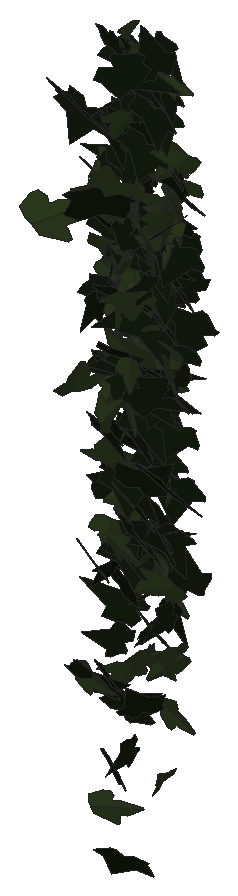
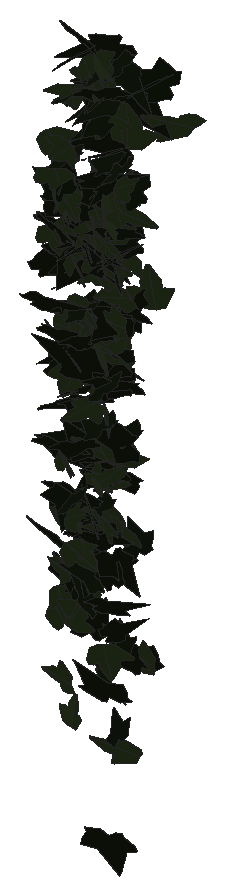
# SketchUp Ruby script. Lengths in millimetres.
U = 1.mm
M = Sketchup.active_model
def pt(a) = Geom::Point3d.new(a.map { |v| v * U })
def face(e, loops, mat)
  f = e.add_face(loops[0].map { |a| pt(a) })
  loops[1..].each { |l| e.add_face(l.map { |a| pt(a) }).erase! }
  f.material = f.back_material = mat if mat
  f
end
# faces: each face lists its corners as indices into pts; further lists are holes
def faces(e, pts, list, mat = nil) = list.each { |f| face(e, (f[0].is_a?(Array) ? f : [f]).map { |l| l.map { |i| pts[i] } }, mat) }
# xy, xz, yz: faces in a plane at the given z, y or x. An outline is a flat list of corners, or four numbers for a rectangle; further outlines are holes
def ring(l) = l.size == 4 ? [[l[0], l[1]], [l[2], l[1]], [l[2], l[3]], [l[0], l[3]]] : l.each_slice(2).to_a
def flat(e, list, mat, &to3) = list.each { |f| face(e, (f[0].is_a?(Array) ? f : [f]).map { |l| ring(l).map { |u, v| to3.(u, v) } }, mat) }
def xy(e, z, list, mat = nil) = flat(e, list, mat) { |x, y| [x, y, z] }
def xz(e, y, list, mat = nil) = flat(e, list, mat) { |x, z| [x, y, z] }
def yz(e, x, list, mat = nil) = flat(e, list, mat) { |y, z| [x, y, z] }
def lines(e, pts, list) = list.each { |a, b| e.add_line(pt(pts[a]), pt(pts[b])) }
# prism: a flat outline (further loops are holes) pulled along v
def prism(e, loops, v, mat = nil)
  f = face(e, loops, mat); d = Geom::Vector3d.new(v.map { |x| x * U })
  f.pushpull(f.normal.samedirection?(d) ? d.length : -d.length)
end
def box(e, o, s, mat = nil) = prism(e, [[o, [o[0] + s[0], o[1], o[2]], [o[0] + s[0], o[1] + s[1], o[2]], [o[0], o[1] + s[1], o[2]]]], [0, 0, s[2]], mat)
def at(x, y, z, deg = 0) = Geom::Transformation.translation(pt([x, y, z])) * Geom::Transformation.rotation(ORIGIN, Z_AXIS, deg.degrees)
def axes(o, x, y, z) = Geom::Transformation.new([*x, 0, *y, 0, *z, 0, *pt(o).to_a, 1])
def part(name) = M.definitions.add(name)
# library, detail: a bought-in or finely detailed component or shape, given as its bounding box
def library(name, o, s) = part(name).tap { |d| box(d.entities, o, s) }
def detail(e, o, s) = box(e.add_group.entities, o, s)
def put(e, d, t, mat = nil) = e.add_instance(d, t).tap { |i| i.material = mat if mat }
def group(e, t, mat = nil) = e.add_group.tap { |g| g.transformation = t; g.material = mat if mat }.entities
root = M.entities
M.materials.add("efeu1").color = [18, 25, 13]
M.materials.add("efeu2").color = [43, 57, 29]
c1 = part("ivyleaf_10")
p = [[0,12.8,-0.8],[-1.5,51.3,-10.9],[-4.9,51,-11.6],[-13.6,26.5,-7.3],[-13.2,15.9,-4.6],[-21.1,19.3,-7.2],
  [-29.5,16.3,-8.3],[-29.2,8.3,-6.2],[-19.7,-9.8,0.5],[-7.6,-13,4],[1,-12.2,5.8],[-0.4,51.1,-11.1],
  [-1.5,51.1,-10.9],[1,-12.4,5.9],[16.9,-12.4,3.5],[35.1,9.1,-5.1],[35,12.9,-6.1],[20.5,16.4,-4.9],
  [15.8,15,-3.8],[15.3,27.6,-7.1],[12.8,31.3,-7.8]]
faces(c1.entities,p,[[0,1,2,3,4,5,6,7,8,9,10],[11,12,0,13,14,15,16,17,18,19,20]],"efeu2")
c2 = part("ivyleaf_9")
p = [[39.1,54.8,31.7],[34.5,51.8,30.2],[-5.3,25.2,17.3],[-17.9,28.3,20.9],[-21.6,21.7,17],[-20.2,4.3,5.3],
  [-22.9,-0.3,2.5],[-17.1,-4,-0.6],[-2,-2.1,-1.2],[-0.7,-15.4,-10.1],[16.6,-22.3,-16.7],[21.1,-15.1,-12.5],
  [32.7,-10.7,-11],[46.1,-1.8,-6.6],[30.8,11.2,3.8]]
faces(c2.entities,p,[[0,1,2,3,4,5,6,7,8,9,10,11,12,13,14]],"efeu1")
put(root,c1,axes([2290.2,709.3,1400.4],[0.97275,0.17788,-1.07304],[1.40084,0.81633,0.48592],[1.52409,-0.86385,0.23824]))
put(root,c2,axes([2377.5,752.5,1448.9],[0.14365,0.58872,-0.9233],[-0.26602,-0.91274,-0.59341],[-2.067,0.15838,0.0122]))
put(root,c1,axes([2316.7,763.5,1090.1],[-0.66136,-1.0008,-0.16593],[-0.09697,-0.15796,1.0594],[-1.92828,0.3512,0.00364]))
put(root,c1,axes([2328.9,817.8,1411.2],[-1.34176,-0.83813,-0.16697],[-0.20573,-0.12726,1.09521],[-1.61342,0.71324,-0.00079]))
put(root,c2,axes([2274.2,837.1,1534],[-0.48902,-0.80421,0.44674],[-0.28635,-0.42086,-0.84415],[1.7273,-0.29745,-0.01347]))
put(root,c2,axes([2235.3,828.8,1548.6],[1.07872,-0.62146,0.50238],[0.63705,-0.37466,-0.8411],[1.38105,0.65824,-0.00442]))
put(root,c1,axes([2334.8,804.3,1022.1],[0.12241,0.13321,-0.95605],[0.36378,0.93744,0.14348],[1.80076,-0.19843,0.03601]))
put(root,c2,axes([2326.3,837.4,1560.7],[-0.62974,0.95802,-0.29231],[0.15978,-0.28024,-1.01348],[-1.89957,-0.34117,0.01166]))
put(root,c2,axes([2366.7,863,493.4],[0.72019,0.24051,0.68698],[-1.11421,-0.3595,0.44833],[0.82312,-0.69706,0.00581]))
put(root,c2,axes([2349.4,859.3,421.6],[-1.05888,0.44266,-0.4062],[0.60519,-0.25276,-0.71098],[-0.97014,-0.64082,-0.00016]))
put(root,c1,axes([2348.7,860,1216.7],[-1.12147,-0.74693,-0.07449],[0.0736,0.06436,-0.95133],[1.42671,-0.59045,-0.00947]))
put(root,c1,axes([2333.5,871.9,1085.7],[1.06286,-0.42346,0.37129],[0.53859,-0.24108,-0.70061],[0.92671,0.62579,-0.01865]))
put(root,c1,axes([2363.2,872.1,590.4],[-0.21119,-0.87133,-0.02569],[0.01241,0.02507,-0.87836],[1.65898,-0.11111,0.0033]))
put(root,c1,axes([2282.6,865.9,295.7],[0.39113,0.02166,-0.78165],[1.47156,0.11491,0.20648],[0.22197,-0.8,0.0085]))
put(root,c2,axes([2317.9,858,1610.1],[0.58229,-0.14445,-0.95844],[0.17653,1.0048,-0.12182],[1.83623,-0.05079,0.31564]))
put(root,c1,axes([2378.9,863.5,1309.6],[0.77263,-0.51903,-0.73941],[-0.23187,0.77177,-0.60864],[1.70363,0.34043,0.2525]))
put(root,c2,axes([2253.3,890,1162.6],[0.00856,-0.01792,-0.78132],[0.86287,-0.63636,0.0172],[-1.21153,-0.45335,0.00673]))
put(root,c1,axes([2404.6,878.2,717.3],[-1.02729,-0.16948,0.65309],[-1.18951,-0.18951,-0.56574],[0.48379,-0.82581,-0.00421]))
put(root,c2,axes([2241.7,892.9,703.3],[-0.13393,-0.33618,0.8001],[0.32971,-0.79201,-0.31754],[1.61846,0.13353,0.1309]))
put(root,c2,axes([2368.5,874.4,1230.9],[-0.93545,0.63087,-0.02799],[0.02173,-0.02658,-0.79971],[-1.20166,-0.49159,0.00733]))
put(root,c2,axes([2359.3,898.2,1531.5],[-0.13824,-0.84154,0.32876],[0.03691,-0.33119,-0.84349],[1.7191,-0.06056,0.04454]))
put(root,c1,axes([2284.5,899.7,1018.9],[-0.31094,-0.46684,0.76473],[0.2287,-0.78174,-0.45155],[1.68979,0.0199,0.20183]))
put(root,c2,axes([2275,897.9,505],[1.03107,-0.44276,-0.44674],[0.67092,-0.27456,0.69962],[-0.9914,-0.64629,0.00884]))
put(root,c1,axes([2262.6,890,1385.7],[0.1354,-0.80053,0.19116],[0.07444,-0.18837,-0.8034],[1.56464,0.07824,0.02168]))
put(root,c2,axes([2239.5,890.7,488.3],[-0.15931,-0.1865,0.8269],[1.22664,-0.55372,-0.05964],[1.04789,0.61982,0.19553]))
put(root,c1,axes([2225.2,890.3,497.6],[-0.01762,-0.057,0.84856],[1.58321,-0.17714,-0.00282],[0.33671,0.82992,0.05767]))
put(root,c2,axes([2277,902.9,343.8],[-0.06898,-0.32301,0.75298],[0.10264,-0.75302,-0.32043],[1.55598,0.03535,0.05452]))
put(root,c1,axes([2284.5,896.7,747.1],[-0.23118,0.13012,-0.78485],[1.0314,-0.56772,-0.17799],[-1.1085,-0.55537,-0.00193]))
put(root,c1,axes([2300.4,907.3,827.4],[-0.21099,0.16475,0.74918],[0.0242,-0.75647,0.16823],[1.45971,0.03636,0.1055]))
put(root,c2,axes([2392.8,897.4,655.4],[-1.1123,0.3954,-0.37179],[0.59571,-0.2008,-0.70558],[-0.84386,-0.66293,-0.00803]))
put(root,c2,axes([2335.5,911.4,1455.8],[-0.51598,-0.78331,0.29293],[-0.04145,-0.30122,-0.82563],[1.59108,-0.26187,0.07348]))
put(root,c1,axes([2369.4,911.1,348.7],[-0.21927,-0.55365,-0.58018],[-0.07713,-0.58136,0.56283],[-1.52433,0.10906,0.05498]))
put(root,c2,axes([2297.6,909.5,857.8],[-0.40594,-0.80961,0.00703],[0.00574,-0.00806,-0.83723],[1.54091,-0.21326,0.00497]))
put(root,c1,axes([2309.6,911.9,1366.2],[0.32646,-0.50151,-0.71944],[0.52097,-0.66584,0.5294],[-1.5857,-0.322,0.02581]))
put(root,c2,axes([2375.7,886.7,1615.5],[-1.4427,0.34514,-0.36247],[-0.64294,0.13257,0.83272],[0.70285,0.82972,0.01772]))
put(root,c2,axes([2358.1,908.7,1527.4],[-0.22273,-0.85653,-0.12764],[0.00103,0.12873,-0.86433],[1.64815,-0.11583,-0.01671]))
put(root,c1,axes([2280,909.5,1335.6],[-0.38244,-0.21076,0.84653],[-1.21884,-0.55424,-0.29001],[1.1274,-0.67068,-0.02636]))
put(root,c2,axes([2231.3,904.6,1384.3],[1.3043,-0.63545,0.17635],[0.2473,-0.11923,-0.93459],[1.23049,0.69753,0.0009]))
put(root,c2,axes([2345.4,887.6,1040.1],[0.43491,-0.12055,-0.89764],[0.14129,0.92515,-0.10535],[1.71793,-0.04557,0.23591]))
put(root,c2,axes([2388.5,899.8,1335.4],[-0.60121,0.83525,-0.38794],[0.23352,-0.3683,-0.89287],[-1.73711,-0.33859,0.01424]))
put(root,c1,axes([2308.2,903.8,987.1],[-0.24658,0.72713,-0.22495],[0.05988,-0.22288,-0.73854],[-1.44735,-0.1331,0.00777]))
put(root,c2,axes([2320.1,899.8,1040.4],[-0.00351,-0.65291,-0.69909],[0.35306,0.68557,-0.64078],[1.78597,-0.13681,0.1253]))
put(root,c2,axes([2283.6,913.5,835.5],[0.74569,-0.7456,0.3233],[0.25868,-0.29373,-0.84214],[1.5249,0.41443,-0.01524]))
put(root,c1,axes([2366.6,905.8,1345.5],[-0.7078,-0.78703,-0.0816],[0.0493,0.078,-0.87041],[1.50509,-0.37267,-0.00986]))
put(root,c2,axes([2338.3,910.8,876.1],[1.20093,-0.48552,0.42101],[0.63121,-0.25935,-0.79617],[1.04759,0.71285,-0.00292]))
put(root,c2,axes([2341.9,925.9,1534.3],[-0.61771,-0.57892,0.63941],[-0.32471,-0.62659,-0.65392],[1.60917,-0.34867,0.1135]))
put(root,c2,axes([2327.2,905.1,857.2],[-0.7208,-0.09053,0.74585],[1.40356,-0.2044,0.34967],[0.27324,0.81114,0.17136]))
put(root,c1,axes([2252.5,924.7,1392.4],[-0.09024,-0.09294,0.88427],[0.2738,-0.87466,-0.08422],[1.66992,0.13839,0.06159]))
put(root,c2,axes([2311,919.5,1347.5],[0.45953,0.25043,0.83541],[-1.05181,-0.62664,0.34758],[1.28405,-0.60293,-0.01426]))
put(root,c1,axes([2325.4,908.5,1006.4],[-1.22852,-0.4203,0.14551],[-0.23618,-0.07608,-0.77027],[0.81288,-0.65731,-0.00389]))
put(root,c2,axes([2366.4,913.1,592.5],[0.5923,-0.6475,0.32196],[-0.26017,0.29151,0.7184],[-1.35144,-0.3399,0.0028]))
put(root,c1,axes([2316.5,896.9,1030.5],[-0.06581,-0.62511,-0.66836],[0.43449,0.6418,-0.61208],[1.68661,-0.18973,0.1316]))
put(root,c2,axes([2297.5,906.4,1302.3],[0.70916,-0.72687,-0.4985],[-0.43835,0.44211,-0.81681],[1.61916,0.43805,-0.0028]))
put(root,c1,axes([2368.2,913,1086.2],[-0.74638,0.76754,-0.43408],[0.37053,-0.38798,-0.86192],[-1.63679,-0.43783,0.00282]))
put(root,c1,axes([2275.5,925.6,1127.6],[-0.34073,0.14378,0.92007],[0.84256,-0.81113,0.2129],[1.55925,0.46972,0.08601]))
put(root,c1,axes([2293.5,913,1492.6],[-0.57424,-0.79982,0.13698],[-0.07739,-0.13106,-0.8548],[1.54244,-0.30434,0.00811]))
put(root,c2,axes([2242.3,920.8,923.9],[0.37381,-0.67069,0.3867],[0.34417,-0.34817,-0.69571],[1.43266,0.25864,0.06623]))
put(root,c2,axes([2364.5,926.4,764.5],[0.55812,-0.67869,-0.44546],[0.42305,-0.3884,0.73809],[-1.48601,-0.36548,0.04282]))
put(root,c2,axes([2314.6,910.5,1064.2],[-1.30419,0.30854,0.21566],[-0.39195,0.06766,-0.75119],[-0.59971,-0.7152,0.02196]))
put(root,c2,axes([2235.2,913.3,1294.1],[1.25785,-0.44203,0.28266],[0.45159,-0.15365,-0.7951],[0.89062,0.70221,0.00395]))
put(root,c1,axes([2250.5,911.1,1255.9],[-1.31377,0.25831,-0.25408],[0.41783,-0.13673,-0.73546],[-0.54859,-0.72275,0.04832]))
put(root,c1,axes([2257.7,915.4,879.2],[-1.23386,-0.40875,-0.10208],[-0.16444,-0.05436,0.76641],[-0.78479,0.65404,-0.0001]))
put(root,c2,axes([2298.5,921.3,768.1],[0.66957,-0.75777,0.28334],[0.27961,-0.244,-0.83496],[1.51411,0.38016,0.02889]))
put(root,c1,axes([2337.9,923.9,730.1],[0.82912,-0.38142,0.66927],[0.92636,-0.45965,-0.57879],[1.13634,0.65302,-0.01649]))
put(root,c2,axes([2256.6,921.2,1616.8],[0.61433,-0.7566,0.18108],[0.13227,-0.16722,-0.82258],[1.47471,0.33018,-0.00166]))
put(root,c1,axes([2294.6,915.8,1234.8],[0.24707,-0.84322,0.02575],[0.00253,-0.02585,-0.85315],[1.60556,0.1298,-0.00262]))
put(root,c1,axes([2275.2,909.2,868],[-0.55152,-0.17322,0.87246],[1.53709,0.33325,0.33442],[-0.70935,0.8568,0.04632]))
put(root,c2,axes([2312.8,920.5,741.8],[-0.72515,-0.63351,-0.36322],[0.42686,0.28837,-0.73823],[1.32263,-0.4404,0.03911]))
put(root,c1,axes([2339,923.4,1349.9],[0.2847,0.15587,-0.75993],[-1.25422,-0.38277,-0.20823],[-0.77891,0.67332,0.05754]))
put(root,c2,axes([2355.8,917.9,782.3],[-0.76045,-0.4007,-0.6967],[1.08668,0.40606,-0.561],[1.07652,-0.69294,0.07414]))
put(root,c2,axes([2319.2,932.6,1351.6],[-0.21073,-0.70925,0.54184],[-0.14571,-0.53643,-0.71782],[1.69242,-0.13449,0.00567]))
put(root,c2,axes([2266.1,911.9,854.8],[1.07359,-0.09914,0.51596],[0.97549,-0.0625,-0.57239],[0.21972,0.76191,0.02018]))
put(root,c2,axes([2344.6,922.5,1255.1],[-0.28886,-0.76253,-0.2035],[0.13448,0.19327,-0.77689],[1.496,-0.16461,0.03054]))
put(root,c2,axes([2276.4,913.2,846.3],[-0.4344,-0.37055,-0.79058],[0.84854,0.65311,-0.43484],[1.42872,-0.50056,0.01788]))
put(root,c1,axes([2307.4,922.8,1212],[0.80491,0.47298,-0.45949],[-0.56616,-0.35032,-0.63441],[-1.12004,0.51698,-0.00952]))
put(root,c1,axes([2380.5,929.3,557.7],[-0.41634,-0.59381,0.66253],[-0.3319,-0.64041,-0.63157],[1.66042,-0.27691,0.03988]))
put(root,c1,axes([2362.9,916.7,538.8],[-1.33352,0.30852,-0.17835],[-0.31619,0.06525,0.76556],[0.60001,0.72007,0.00704]))
put(root,c2,axes([2271.2,928.9,651.6],[-0.06364,-0.04847,0.86819],[0.53647,-0.82252,-0.03507],[1.56554,0.27988,0.04731]))
put(root,c1,axes([2385.9,918.4,582.1],[-0.38661,-0.85894,-0.02665],[0.01553,0.02546,-0.88263],[1.63545,-0.20329,0.00208]))
put(root,c2,axes([2323.9,915.9,584.7],[0.1999,0.7706,0.41637],[-0.10302,-0.41284,0.77773],[1.66382,-0.11814,-0.00187]))
put(root,c1,axes([2310.2,918.8,1067.2],[-1.45372,0.09156,-0.56397],[-1.0675,0.05912,0.76927],[0.20706,0.94763,0.00649]))
put(root,c1,axes([2248.6,923.2,753.7],[1.29905,-0.389,0.246],[0.40099,-0.12712,-0.7856],[0.77879,0.71431,-0.00584]))
put(root,c2,axes([2272.2,930.7,550.2],[-0.16902,-0.05871,0.77051],[-1.17088,-0.46393,-0.10626],[0.8899,-0.62156,0.00653]))
put(root,c1,axes([2368.4,924.9,1336.8],[0.85176,0.23412,-0.66488],[-1.13482,-0.2943,-0.50499],[-0.7155,0.74548,0.00945]))
put(root,c2,axes([2257.9,917.7,1058.6],[1.15008,-0.22546,0.53768],[0.97639,-0.1623,-0.64464],[0.52722,0.79242,0.02095]))
put(root,c2,axes([2329.4,924.6,973.2],[-0.38524,-0.84849,-0.34592],[0.11218,0.34147,-0.87206],[1.74028,-0.20984,-0.02036]))
put(root,c2,axes([2306.2,927.1,727.8],[-1.0432,-0.70434,-0.32675],[0.38149,0.25805,-0.89249],[1.42763,-0.58363,-0.00027]))
put(root,c2,axes([2386.9,926.4,1285],[-1.4346,-0.27842,-0.31916],[0.5736,0.10515,-0.80354],[0.56634,-0.81178,0.00538]))
put(root,c2,axes([2313.5,932.8,1141],[-0.03816,-0.14138,-0.81916],[-0.29271,-0.80463,0.14263],[-1.55477,0.15495,-0.00675]))
put(root,c1,axes([2357.5,922.9,1282.7],[-1.24112,-0.34574,0.33267],[-0.4648,-0.24399,-0.73232],[0.78601,-0.69022,0.09224]))
put(root,c2,axes([2333.1,925.3,1142],[-0.4727,-0.83847,-0.37533],[0.21964,0.35724,-0.87444],[1.7345,-0.27374,0.00844]))
put(root,c1,axes([2296.4,932.3,841.6],[0.21175,-0.72273,0.55876],[0.25911,-0.54348,-0.73008],[1.71923,0.17093,0.04122]))
put(root,c1,axes([2391.5,930.2,1441.7],[-0.82374,-0.59665,0.54528],[-0.44006,-0.50129,-0.73205],[1.47403,-0.48308,0.08618]))
put(root,c1,axes([2284,918.3,1362.9],[0.02125,-0.84532,-0.23235],[-0.0132,0.23227,-0.84539],[1.66843,0.01261,-0.00373]))
put(root,c1,axes([2369.6,931.3,1325.2],[0.43804,-0.74794,0.4424],[0.29395,-0.41515,-0.78224],[1.62752,0.27629,0.02221]))
put(root,c2,axes([2352.4,921.2,1234.6],[0.08079,0.13758,-0.7754],[-1.23363,-0.4349,-0.11265],[-0.85119,0.64336,0.08967]))
put(root,c1,axes([2352.9,920,735.1],[-0.07431,0.78379,-0.08296],[-0.00463,-0.08318,-0.78474],[-1.50004,-0.03857,0.00653]))
put(root,c1,axes([2318,918.5,748.7],[-1.25979,-0.01059,-0.40762],[0.77554,0.01078,-0.66201],[0.02791,-0.7773,-0.00363]))
put(root,c2,axes([2250.8,923.5,1028.4],[1.19364,-0.3592,0.49894],[0.82697,-0.24524,-0.72275],[0.82776,0.76298,0.00258]))
put(root,c2,axes([2335.1,921.6,1261.2],[0.37904,-0.65973,-0.36905],[-0.21447,0.35147,-0.68911],[1.42263,0.22876,-0.00556]))
put(root,c1,axes([2295.1,913.2,952.2],[0.24235,-0.50966,-0.57524],[-0.23692,0.56171,-0.52522],[1.44338,0.17777,0.01037]))
put(root,c2,axes([2303.4,928.2,737.7],[0.00018,0.50919,0.71944],[-0.1297,-0.71728,0.50767],[1.67246,-0.05568,0.03929]))
put(root,c2,axes([2377.9,928.9,871],[-1.20889,-0.44885,-0.39356],[0.60771,0.23008,-0.77777],[0.95993,-0.71092,-0.00324]))
put(root,c1,axes([2374.8,921.5,1090.6],[-0.25057,0.03384,-0.79601],[-1.48575,0.15573,0.13574],[0.30298,0.79165,0.00733]))
put(root,c2,axes([2397.9,908.6,1054.8],[-0.40755,0.63683,0.54638],[-0.32186,0.51956,-0.67186],[-1.5642,-0.27284,-0.00411]))
put(root,c1,axes([2283.5,923.8,1293.4],[-1.55723,-0.40103,0.29579],[0.52191,0.11244,0.91102],[-0.79188,0.86274,0.01876]))
put(root,c1,axes([2377.9,918.1,1375.3],[-0.90889,0.63249,0.08716],[-0.11203,0.06476,-0.79249],[-1.20995,-0.48111,0.00791]))
put(root,c1,axes([2371.1,936,1284.7],[-0.2024,-0.53862,0.60657],[0.35162,-0.61177,-0.51084],[1.50329,0.07057,0.20116]))
put(root,c1,axes([2307.3,921.5,1603.1],[1.04107,-0.58497,-0.26484],[-0.27264,0.22798,-0.79941],[1.19131,0.56337,0.04849]))
put(root,c1,axes([2301.3,925.2,1570.1],[-0.00161,-0.92422,-0.0039],[-0.00202,0.0039,-0.92422],[1.759,-0.00084,-0.00107]))
put(root,c1,axes([2331.3,924.9,730.6],[0.13885,-0.88071,-0.02433],[-0.00284,0.02429,-0.88373],[1.6768,0.07297,0.00052]))
put(root,c2,axes([2306.3,932.8,1581.1],[0.2962,-0.81555,0.1224],[0.15187,-0.10908,-0.82829],[1.56218,0.16524,0.05731]))
put(root,c2,axes([2269.7,924.3,693.3],[-0.18862,0.68835,-0.5205],[0.15979,-0.51374,-0.69541],[-1.63465,-0.12965,-0.00792]))
put(root,c2,axes([2361.2,937.7,1020.9],[-0.04632,-0.4959,0.68379],[0.52803,-0.65081,-0.46211],[1.51839,0.21119,0.18156]))
put(root,c1,axes([2256.4,928.6,1239.6],[-0.78871,0.49964,-0.41549],[0.27797,-0.40856,-0.63699],[-1.2051,-0.42125,0.125]))
put(root,c1,axes([2351.5,936.5,1333.2],[0.1494,-0.55553,0.59073],[0.56955,-0.53176,-0.53984],[1.4344,0.269,0.15282]))
put(root,c2,axes([2285,936.7,933.6],[0.32248,-0.75782,0.35446],[0.24364,-0.33392,-0.77508],[1.5735,0.20701,0.04737]))
put(root,c2,axes([2358.9,938.6,1219.3],[0.34166,-0.61811,0.57461],[0.38808,-0.5383,-0.64274],[1.5586,0.26953,0.03408]))
put(root,c1,axes([2273,916,1135.8],[0.3903,0.09961,-0.82729],[1.43213,0.3438,0.22793],[0.68116,-0.77991,-0.00518]))
put(root,c1,axes([2272.9,933,1135.4],[0.71532,-0.57183,0.34634],[0.45988,-0.25427,-0.68203],[1.18635,0.44336,0.05555]))
put(root,c2,axes([2261,931.6,1169],[-1.10938,-0.53277,-0.42244],[0.57877,0.29339,-0.78963],[1.15739,-0.65738,-0.01005]))
put(root,c2,axes([2291.5,942.6,1532.3],[-0.69229,-0.5854,0.46056],[0.00593,-0.51374,-0.65053],[1.4176,-0.28373,0.22764]))
put(root,c1,axes([2369.3,941.2,851.2],[-0.08443,-0.10074,0.81796],[0.57002,-0.7651,-0.07798],[1.46125,0.29264,0.07768]))
put(root,c2,axes([2254.8,937.2,1237.6],[-0.44311,0.02472,-0.74149],[1.15896,-0.43756,-0.20579],[-0.80656,-0.64231,0.11166]))
put(root,c2,axes([2340.8,914,692.8],[0.15751,-0.1459,0.76396],[0.31083,0.7544,0.12638],[-1.44724,0.14615,0.11029]))
put(root,c1,axes([2284.6,928,512],[-0.9658,-0.6926,0.08549],[-0.08213,-0.07435,-0.85856],[1.32562,-0.50921,0.00909]))
put(root,c2,axes([2273.3,928.8,1479.3],[-0.40363,-0.05665,-0.91189],[1.61799,0.33069,-0.21826],[0.63698,-0.87588,-0.02342]))
put(root,c2,axes([2238.7,922.8,1157],[0.57973,0.20191,-0.67109],[1.01881,0.40522,0.3649],[0.86079,-0.61558,0.02009]))
put(root,c2,axes([2245.9,939.9,1277.7],[-0.18538,-0.86981,0.11578],[-0.01928,-0.11537,-0.87524],[1.66991,-0.09789,0.00275]))
put(root,c2,axes([2360.3,937.6,641.5],[-0.22602,-0.07689,-0.80535],[1.51177,-0.16548,-0.10134],[-0.29206,-0.79707,0.09872]))
put(root,c1,axes([2342.9,927.4,1092.2],[-0.37324,0.02326,0.77628],[-1.47104,-0.08384,-0.19275],[0.14399,-0.79626,0.04297]))
put(root,c1,axes([2344.6,926.6,1131.5],[-0.61895,-0.69186,-0.17785],[0.18472,0.1508,-0.76413],[1.34694,-0.33861,0.02307]))
put(root,c2,axes([2294.1,931.3,1270.9],[-0.38004,0.63241,-0.49087],[0.11643,-0.49237,-0.65924],[-1.51917,-0.19594,0.07227]))
put(root,c2,axes([2385.3,921.6,1412],[0.25113,0.04339,-0.81934],[-1.55703,0.07003,-0.12804],[0.11868,0.82693,0.05383]))
put(root,c2,axes([2333.5,921.3,1214.5],[-0.31261,0.3405,0.69057],[-0.94706,0.49188,-0.36089],[-1.11822,-0.51178,0.1126]))
put(root,c2,axes([2342.4,942.9,1195.3],[-0.23993,-0.79959,0.20005],[0.00575,-0.20282,-0.80877],[1.56868,-0.12155,0.03356]))
put(root,c2,axes([2232.3,932.2,922.2],[0.52151,0.08156,-0.79711],[1.48811,0.15691,0.28484],[0.33331,-0.82816,-0.02453]))
put(root,c1,axes([2332.4,940.2,1234.8],[-0.69405,-0.56042,0.50547],[-0.17781,-0.52355,-0.64787],[1.4253,-0.33821,0.16532]))
put(root,c1,axes([2288.5,925.2,1341.7],[0.31425,-0.75649,-0.37081],[0.00207,0.37806,-0.77079],[1.60342,0.14778,0.07367]))
put(root,c1,axes([2307.9,921.9,1123.2],[0.12819,0.69163,0.36124],[0.0871,0.35846,-0.69483],[-1.48248,0.08086,-0.00959]))
put(root,c2,axes([2277.2,929.7,434.3],[-0.5695,0.15401,0.72475],[1.18101,-0.37501,0.33589],[0.77055,0.6886,0.02083]))
put(root,c1,axes([2284.4,933.4,832.9],[0.79573,0.66594,0.37045],[-0.38832,-0.30928,0.78627],[1.39736,-0.46517,0.00755]))
put(root,c1,axes([2383.9,932.9,1268.4],[-1.21834,-0.52196,0.17914],[-0.25354,-0.12008,-0.82593],[1.01921,-0.65381,0.00868]))
put(root,c2,axes([2307.2,945.3,1396.8],[-0.60467,-0.72583,-0.52401],[-0.29999,-0.50199,0.79089],[-1.67716,0.35147,0.04745]))
put(root,c1,axes([2317.5,934.8,1581.1],[1.45144,-0.35159,-0.01271],[-0.0131,0.01542,-0.8397],[0.66945,0.76258,0.01112]))
put(root,c2,axes([2260.4,928.8,1403.5],[0.30017,-0.65442,-0.58031],[-0.29575,0.55932,-0.67298],[1.63815,0.22089,-0.01517]))
put(root,c2,axes([2260.6,939.5,1315.3],[-0.74058,-0.69537,-0.25303],[0.23174,0.22181,-0.79684],[1.38912,-0.40773,-0.00196]))
put(root,c1,axes([2258.9,945.1,1333.7],[0.21369,-0.51871,0.57243],[0.28492,-0.55287,-0.53035],[1.44232,0.18606,0.01996]))
put(root,c2,axes([2241.6,947.2,1433.5],[0.14173,-0.7399,0.40506],[0.05845,-0.40398,-0.74359],[1.60432,0.08008,-0.00869]))
put(root,c2,axes([2320.7,918.1,1536.2],[0.25814,-0.12002,-0.95271],[-1.30435,0.66184,-0.18094],[1.28006,0.6986,0.00775]))
put(root,c2,axes([2260.7,948.8,1258],[-0.39907,-0.564,0.47955],[-0.33574,-0.44599,-0.60167],[1.36838,-0.27391,-0.00777]))
put(root,c2,axes([2359.6,921.4,773.1],[0.68162,0.70014,0.06005],[0.05005,0.054,-0.78642],[-1.33645,0.35911,0.00118]))
put(root,c2,axes([2339.5,947.5,1547.2],[-0.00054,-0.75848,0.35794],[0.12724,-0.35682,-0.75606],[1.59113,0.02828,0.06058]))
put(root,c2,axes([2373.9,947.1,956.3],[-0.63231,-0.66755,0.21984],[-0.16623,-0.20207,-0.74557],[1.32724,-0.34334,0.01135]))
put(root,c2,axes([2284.2,938.6,1604.9],[0.78699,-0.7399,-0.03157],[-0.02502,0.02882,-0.8476],[1.40924,0.41371,0.00258]))
put(root,c2,axes([2366.1,931.3,1331.3],[0.44107,0.36283,-0.66877],[-1.08167,-0.38224,-0.40433],[-0.96273,0.59569,0.14789]))
put(root,c1,axes([2283.8,934.3,1242],[-1.38179,-0.29018,0.16338],[-0.26709,-0.08877,-0.78131],[0.57476,-0.73887,0.02971]))
put(root,c1,axes([2312.1,941.7,1611.2],[-0.12133,-0.80108,0.27625],[0.23175,-0.28281,-0.79202],[1.59599,-0.01983,0.13601]))
put(root,c2,axes([2329.2,949.1,997.1],[-0.54328,-0.71382,0.21623],[-0.0961,-0.2125,-0.76816],[1.41625,-0.28825,0.03082]))
put(root,c2,axes([2347.4,927.1,1296.9],[0.1481,-0.05125,-0.83119],[-1.51815,0.23516,-0.08918],[0.45517,0.80102,-0.027]))
put(root,c1,axes([2238.5,936.5,1196.8],[0.75147,-0.03108,0.66099],[1.24758,0.12348,-0.38577],[-0.17197,0.75997,0.08971]))
put(root,c2,axes([2257.2,942.5,1033.4],[-0.77387,-0.63217,-0.4158],[0.45348,0.34104,-0.75152],[1.3668,-0.47108,0.01392]))
put(root,c1,axes([2359,944,858.6],[0.86918,-0.62733,0.2177],[0.24383,-0.17601,-0.77596],[1.24003,0.47432,-0.00001]))
put(root,c1,axes([2279.1,947.1,1630.6],[0.13478,-0.76777,0.36554],[0.10108,-0.36209,-0.77083],[1.61523,0.08672,0.01774]))
put(root,c2,axes([2335.2,953.2,783],[0.11416,-0.71944,0.45891],[0.02301,-0.45928,-0.7216],[1.62392,0.05708,-0.02204]))
put(root,c2,axes([2335.4,953,1254.5],[-0.35695,-0.67235,0.37039],[-0.22499,-0.35144,-0.69781],[1.44352,-0.22103,-0.01717]))
put(root,c2,axes([2397.8,951.1,1204.3],[-0.06195,-0.02825,0.82963],[-1.29948,-0.47128,-0.04284],[0.89851,-0.68354,-0.00475]))
put(root,c2,axes([2272.7,933.8,170.9],[0.86835,0.36643,-0.511],[-0.80424,-0.28885,-0.58444],[-0.88622,0.62118,0.02967]))
put(root,c2,axes([2313.1,924.5,644.5],[-0.19823,0.73094,-0.26665],[-0.06911,0.26417,0.73832],[1.47919,0.1103,-0.00124]))
put(root,c1,axes([2286.2,942.1,1080.2],[0.4791,-0.71675,0.0603],[0.03612,-0.05724,-0.75968],[1.36847,0.25245,-0.00106]))
put(root,c2,axes([2345.5,952.4,1425.2],[0.08906,-0.72136,0.40497],[0.22727,-0.39548,-0.71826],[1.55796,0.09893,0.08162]))
put(root,c2,axes([2309,950.6,1154.8],[0.50281,-0.79338,0.35827],[0.28691,-0.32705,-0.83541],[1.63174,0.30198,0.03649]))
put(root,c2,axes([2281.8,946.4,739.4],[-0.87803,-0.61749,-0.21894],[0.25793,0.17203,-0.77078],[1.21991,-0.48081,0.00539]))
put(root,c2,axes([2335.3,945.6,893.6],[-0.5348,-0.73455,-0.21787],[0.10029,0.21298,-0.78604],[1.45475,-0.28472,-0.0259]))
put(root,c2,axes([2308.1,940,1039.3],[0.32196,-0.274,0.85823],[1.59522,-0.27226,-0.25214],[0.62859,0.83129,0.20029]))
put(root,c2,axes([2291.5,934.6,1550.5],[0.96776,-0.54488,-0.44211],[-0.41967,0.39424,-0.73951],[1.26778,0.54644,0.09268]))
put(root,c2,axes([2283.2,944.1,606.4],[-1.07136,-0.4876,-0.29346],[-0.3744,-0.22061,0.7439],[-1.01634,0.59526,0.03531]))
put(root,c1,axes([2336,943.4,1233.6],[0.73884,-0.70909,0.03542],[0.01885,-0.03496,-0.80837],[1.3511,0.38825,-0.00809]))
put(root,c2,axes([2329.1,942.6,1624.1],[0.40535,-0.76786,-0.27667],[-0.09901,0.27259,-0.79656],[1.55021,0.21819,0.02147]))
put(root,c2,axes([2329.6,931.6,1245.1],[1.68944,0.19627,-0.27277],[-0.50576,-0.06161,-0.90912],[-0.39148,0.9266,-0.00267]))
put(root,c1,axes([2354,950,651.5],[-0.28879,0.09264,-0.72431],[0.76415,-0.60734,-0.16179],[-1.16081,-0.42285,0.07369]))
put(root,c1,axes([2277.4,933.4,1285.8],[-0.32902,0.69239,0.3044],[-0.37958,0.25946,-0.70345],[-1.38853,-0.23499,0.12018]))
put(root,c1,axes([2303,934.6,1311.1],[0.25866,-0.68549,-0.46636],[-0.06354,0.46768,-0.69716],[1.57665,0.13131,0.04841]))
put(root,c1,axes([2342.2,943.4,1556.1],[1.19117,0.55172,-0.09423],[-0.14899,-0.05367,-0.83426],[-1.05477,0.63065,0.01143]))
put(root,c1,axes([2364.1,947.5,1353.2],[0.04793,-0.77462,0.1506],[-0.02672,-0.15109,-0.77481],[1.50162,0.02204,-0.01859]))
put(root,c1,axes([2343,932.4,1146.1],[0.34108,-0.14057,-0.81291],[-0.9892,0.62677,-0.22297],[1.21929,0.54781,0.04651]))
put(root,c1,axes([2349.1,947.1,1348.2],[-0.28445,-0.75542,0.15525],[-0.01935,-0.1562,-0.7698],[1.46763,-0.14847,0.01994]))
put(root,c2,axes([2278.4,953,1577.8],[-0.83066,-0.74024,-0.11235],[0.09883,0.09981,-0.85931],[1.42154,-0.43949,-0.00591]))
put(root,c1,axes([2331.3,959.5,759.6],[-0.07125,-0.12912,0.80787],[0.32477,-0.79216,-0.1187],[1.5228,0.1629,0.06312]))
put(root,c1,axes([2299.9,940.4,1307],[-0.73567,-0.61967,-0.34452],[0.62238,0.19234,-0.71286],[1.19727,-0.48074,0.15888]))
put(root,c2,axes([2363.2,951,1097.3],[-1.24584,-0.35747,-0.23831],[0.38994,0.12202,-0.7458],[0.7187,-0.68586,-0.00847]))
put(root,c2,axes([2249.1,953.8,1452.8],[0.5324,-0.74988,0.2179],[0.13337,-0.20642,-0.80033],[1.48021,0.28831,-0.00626]))
put(root,c1,axes([2310.3,934,967.8],[-0.49155,-0.42652,-0.70004],[0.91865,0.5141,-0.49132],[1.26099,-0.54079,0.08505]))
put(root,c2,axes([2266,958.1,1466.9],[-0.46039,-0.76392,0.18614],[0.02623,-0.19884,-0.79813],[1.49621,-0.23157,0.07127]))
put(root,c2,axes([2399.7,931.4,691.7],[-1.57981,0.44308,-0.2176],[-0.37022,0.09766,0.94092],[0.86344,0.85255,0.00531]))
put(root,c1,axes([2362.6,934.5,1353.6],[-0.06923,-0.51541,-0.59691],[0.26914,0.5836,-0.51253],[1.4766,-0.13054,0.06544]))
put(root,c1,axes([2345.2,951.9,446.9],[0.19406,-0.05267,0.80903],[1.46097,-0.25606,-0.11342],[0.49641,0.77418,0.01753]))
put(root,c2,axes([2322.5,939.3,1265.5],[-0.61858,0.35882,0.61035],[-0.96509,0.35071,-0.47621],[-0.94038,-0.59596,0.08724]))
put(root,c1,axes([2340.8,941.5,1022.7],[-1.26496,-0.46754,-0.22362],[0.33405,0.1391,-0.81253],[0.92808,-0.68732,-0.01233]))
put(root,c1,axes([2352.4,947.3,1443.4],[-1.13188,0.41409,-0.37892],[0.50641,-0.2781,-0.72153],[-0.9406,-0.64803,0.06751]))
put(root,c1,axes([2257.5,948.1,1279.2],[1.15788,-0.315,-0.53264],[0.93319,-0.21029,0.68441],[-0.71847,-0.78078,0.03055]))
put(root,c1,axes([2329.3,955.7,701.7],[-0.57757,-0.61715,0.51894],[-0.3353,-0.49033,-0.68615],[1.49754,-0.34781,0.04651]))
put(root,c2,axes([2351.4,957.3,1364.7],[0.3036,-0.47445,0.62182],[0.65149,-0.52827,-0.49088],[1.33846,0.36475,0.09789]))
put(root,c1,axes([2234.4,952.6,1153.2],[0.20515,-0.17311,0.79881],[1.50196,-0.1877,-0.14717],[0.40494,0.78389,0.14117]))
put(root,c2,axes([2258,963.6,1025.4],[-0.03146,-0.63699,0.61836],[0.09358,-0.61818,-0.63549],[1.68701,0.02241,0.04678]))
put(root,c2,axes([2302.3,955.1,1107.7],[-0.54577,-0.81797,-0.1913],[0.13638,0.17758,-0.86674],[1.59294,-0.29546,0.00866]))
put(root,c2,axes([2245.2,940.3,1158.9],[1.43316,0.05984,-0.12105],[-0.22905,-0.01367,-0.75539],[-0.11657,0.76257,-0.00404]))
put(root,c1,axes([2273.4,950,772.4],[1.15152,-0.49393,0.00823],[0.01209,-0.00524,-0.78106],[0.9401,0.60508,-0.00004]))
put(root,c2,axes([2272.2,935.6,1553.1],[1.43569,-0.07109,-0.35592],[-0.53493,0.40497,-0.6766],[0.43705,0.7292,0.34106]))
put(root,c2,axes([2270.1,942.7,1518.5],[1.25134,-0.42141,-0.2776],[-0.29015,0.26875,-0.76907],[0.91552,0.66116,0.13568]))
put(root,c1,axes([2372.8,948.3,1386.6],[-1.40447,-0.28634,0.22004],[-0.35588,-0.12528,-0.79014],[0.58796,-0.7598,0.04736]))
put(root,c2,axes([2379.8,953.5,1294.8],[-1.29412,0.05996,-0.41279],[0.77879,-0.05723,-0.68237],[-0.15398,-0.7934,0.01802]))
put(root,c2,axes([2409.6,948.1,1134.6],[-1.36125,-0.34201,-0.38711],[-0.66808,-0.16323,0.7928],[-0.72121,0.79673,-0.00375]))
